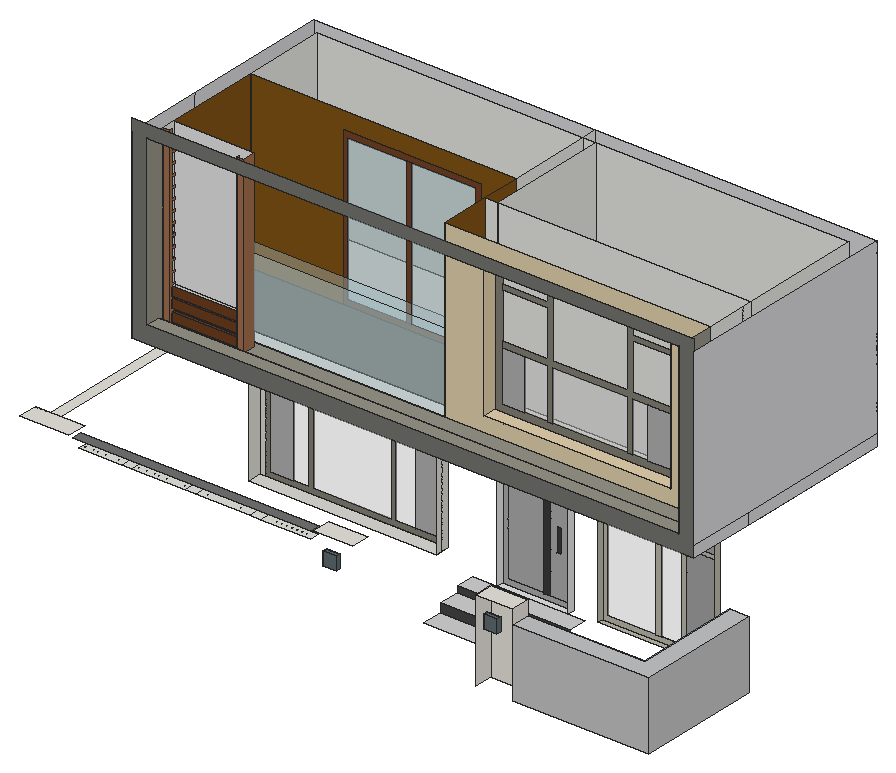
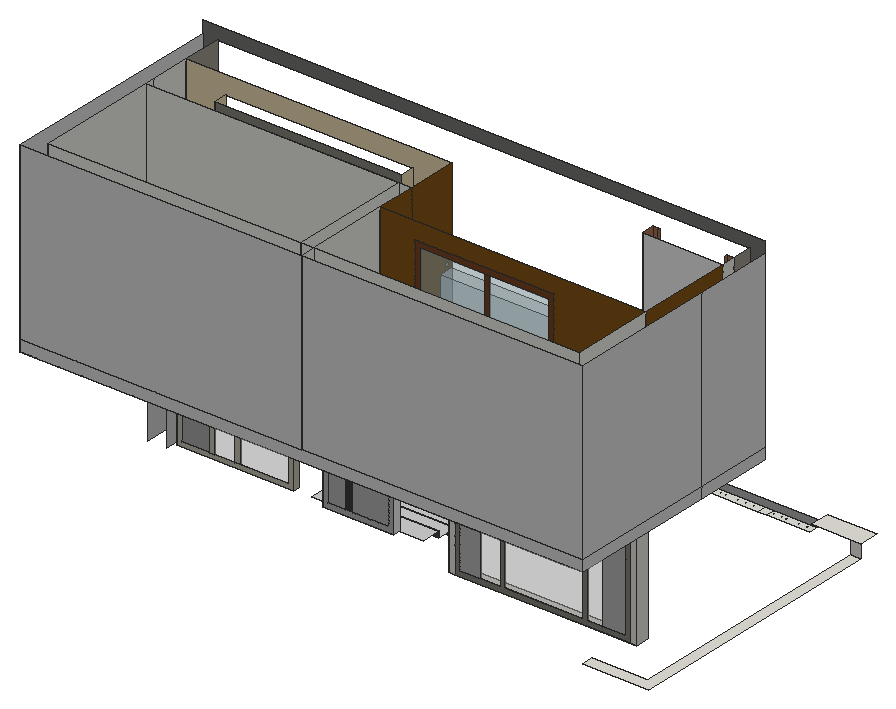
# SketchUp Ruby script. Lengths in inches.
U = 1.inch
M = Sketchup.active_model
def pt(a) = Geom::Point3d.new(a.map { |v| v * U })
def face(e, loops, mat)
  f = e.add_face(loops[0].map { |a| pt(a) })
  loops[1..].each { |l| e.add_face(l.map { |a| pt(a) }).erase! }
  f.material = f.back_material = mat if mat
  f
end
# faces: each face lists its corners as indices into pts; further lists are holes
def faces(e, pts, list, mat = nil) = list.each { |f| face(e, (f[0].is_a?(Array) ? f : [f]).map { |l| l.map { |i| pts[i] } }, mat) }
# xy, xz, yz: faces in a plane at the given z, y or x. An outline is a flat list of corners, or four numbers for a rectangle; further outlines are holes
def ring(l) = l.size == 4 ? [[l[0], l[1]], [l[2], l[1]], [l[2], l[3]], [l[0], l[3]]] : l.each_slice(2).to_a
def flat(e, list, mat, &to3) = list.each { |f| face(e, (f[0].is_a?(Array) ? f : [f]).map { |l| ring(l).map { |u, v| to3.(u, v) } }, mat) }
def xy(e, z, list, mat = nil) = flat(e, list, mat) { |x, y| [x, y, z] }
def xz(e, y, list, mat = nil) = flat(e, list, mat) { |x, z| [x, y, z] }
def yz(e, x, list, mat = nil) = flat(e, list, mat) { |y, z| [x, y, z] }
def lines(e, pts, list) = list.each { |a, b| e.add_line(pt(pts[a]), pt(pts[b])) }
# prism: a flat outline (further loops are holes) pulled along v
def prism(e, loops, v, mat = nil)
  f = face(e, loops, mat); d = Geom::Vector3d.new(v.map { |x| x * U })
  f.pushpull(f.normal.samedirection?(d) ? d.length : -d.length)
end
def box(e, o, s, mat = nil) = prism(e, [[o, [o[0] + s[0], o[1], o[2]], [o[0] + s[0], o[1] + s[1], o[2]], [o[0], o[1] + s[1], o[2]]]], [0, 0, s[2]], mat)
def at(x, y, z, deg = 0) = Geom::Transformation.translation(pt([x, y, z])) * Geom::Transformation.rotation(ORIGIN, Z_AXIS, deg.degrees)
def axes(o, x, y, z) = Geom::Transformation.new([*x, 0, *y, 0, *z, 0, *pt(o).to_a, 1])
def part(name) = M.definitions.add(name)
# library, detail: a bought-in or finely detailed component or shape, given as its bounding box
def library(name, o, s) = part(name).tap { |d| box(d.entities, o, s) }
def detail(e, o, s) = box(e.add_group.entities, o, s)
def put(e, d, t, mat = nil) = e.add_instance(d, t).tap { |i| i.material = mat if mat }
def group(e, t, mat = nil) = e.add_group.tap { |g| g.transformation = t; g.material = mat if mat }.entities
root = M.entities
M.materials.add("[Blinds Vertical Pattern]").color = [212, 212, 214]
M.materials.add("[Blinds Vertical Stripe Gray]").color = [160, 160, 160]
M.materials.add("[Blinds Vertical Stripe Gray]1").color = [175, 175, 175]
M.materials.add("[Blinds Weave]").color = [127, 82, 22]
M.materials.add("[Carpet Diamond Olive]").color = [87, 77, 61]
M.materials.add("[Carrera Marble]").color = [207, 207, 207]
M.materials.add("[Color M01]").color = [226, 226, 226]
M.materials.add("[Color M03]").color = [170, 170, 170]
M.materials.add("[Color M05]").color = [114, 114, 114]
M.materials.add("[Color M07]").color = [58, 58, 58]
M.materials.add("[Concrete Block 8x8 Gray]").color = [114, 114, 111]
M.materials.add("[Fencing Metal Straight]").color = [194, 195, 196]
M.materials.add("[Formica Graystone]").color = [186, 182, 168]
M.materials.add("[Formica Graystone]2").color = [130, 127, 117]
M.materials.add("[Formica Graystone]3").color = [149, 146, 135]
M.materials.add("[Formica Speckled Grey]").color = [94, 105, 111]
M.materials.add("[Granite Dark Gray]").color = [69, 68, 68]
M.materials.add("[Quartz Light Brown]").color = [224, 207, 171]
M.materials.add("[Quartz Light Brown]1").color = [199, 184, 152]
M.materials.add("[Terrazzo Tile Light]").color = [219, 217, 210]
M.materials.add("[Tile Travertine 2 inch]").color = [229, 225, 218]
M.materials.add("[Translucent Glass Gray]").color = [226, 226, 226]
M.materials["[Translucent Glass Gray]"].alpha = 0.5
M.materials.add("[Translucent Glass Gray]1").color = [224, 224, 224]
M.materials["[Translucent Glass Gray]1"].alpha = 0.5
M.materials.add("[Translucent Glass Safety]").color = [179, 206, 214]
M.materials["[Translucent Glass Safety]"].alpha = 0.5
M.materials.add("[Translucent Glass Safety]1").color = [204, 235, 244]
M.materials["[Translucent Glass Safety]1"].alpha = 0.38
M.materials.add("[Wood Cherry Original]").color = [107, 60, 29]
M.materials.add("[Wood Veneer 01]").color = [114, 66, 35]
M.materials.add("[Wood Veneer 02]").color = [160, 108, 76]
xy(root,20.25,[[445.64,200.28,587.08,226.75]],"[Carrera Marble]")
xy(root,31.375,[[445.64,226.75,587.08,253.22]],"[Carrera Marble]")
xy(root,38.0625,[[151.04,291.34,388.47,309.84]],"[Terrazzo Tile Light]")
xy(root,39.19,[[445.64,253.22,587.08,277.72]],"[Carrera Marble]")
xy(root,39.19,[[476.45,277.72,566.07,286.22]],"[Color M01]")
xy(root,43.13,[[604.02,277.72,751.39,284.78]],"[Formica Graystone]")
xy(root,102.5625,[[387.01,114.53,403.76,119.71],[590.2,114.53,606.95,119.71]],"[Formica Speckled Grey]")
xy(root,116.1875,[[622.67,119.71,793.87,119.71,793.87,277.72,769.95,277.72,769.95,143.63,622.67,143.63]],"[Fencing Metal Straight]")
xy(root,116.1875,[[0,143.63,12.5625,143.63,12.5625,464.52,83.3125,464.52,83.3125,479.71,0,479.71]],"[Tile Travertine 2 inch]")
xy(root,119.3125,[[387.01,114.53,403.76,119.71],[590.2,114.53,606.95,119.71]],"[Formica Speckled Grey]")
xy(root,119.59,[[[69.95,125.1875,124.17,137.375],[119.99,129.51,120.39,129.56,120.77,129.72,121.09,129.97,121.34,130.29,121.5,130.67,121.55,131.07,121.5,131.48,121.34,131.86,121.09,132.18,120.77,132.43,120.39,132.58,119.99,132.64,119.59,132.58,119.21,132.43,118.88,132.18,118.64,131.86,118.48,131.48,118.43,131.07,118.48,130.67,118.64,130.29,118.88,129.97,119.21,129.72,119.59,129.56],[115.49,129.51,115.89,129.56,116.27,129.72,116.59,129.97,116.84,130.29,117,130.67,117.05,131.07,117,131.48,116.84,131.86,116.59,132.18,116.27,132.43,115.89,132.58,115.49,132.64,115.09,132.58,114.71,132.43,114.38,132.18,114.14,131.86,113.98,131.48,113.93,131.07,113.98,130.67,114.14,130.29,114.38,129.97,114.71,129.72,115.09,129.56],[110.11,129.51,110.52,129.56,110.9,129.72,111.22,129.97,111.47,130.29,111.625,130.67,111.68,131.07,111.625,131.48,111.47,131.86,111.22,132.18,110.9,132.43,110.52,132.58,110.11,132.64,109.71,132.58,109.33,132.43,109.01,132.18,108.76,131.86,108.61,131.48,108.55,131.07,108.61,130.67,108.76,130.29,109.01,129.97,109.33,129.72,109.71,129.56],[104.36,129.51,104.77,129.56,105.15,129.72,105.47,129.97,105.72,130.29,105.875,130.67,105.93,131.07,105.875,131.48,105.72,131.86,105.47,132.18,105.15,132.43,104.77,132.58,104.36,132.64,103.96,132.58,103.58,132.43,103.26,132.18,103.01,131.86,102.86,131.48,102.8,131.07,102.86,130.67,103.01,130.29,103.26,129.97,103.58,129.72,103.96,129.56],[98.93,129.51,99.33,129.56,99.71,129.72,100.03,129.97,100.28,130.29,100.4375,130.67,100.49,131.07,100.4375,131.48,100.28,131.86,100.03,132.18,99.71,132.43,99.33,132.58,98.93,132.64,98.52,132.58,98.15,132.43,97.82,132.18,97.57,131.86,97.42,131.48,97.36,131.07,97.42,130.67,97.57,130.29,97.82,129.97,98.15,129.72,98.52,129.56],[93.43,129.51,93.83,129.56,94.21,129.72,94.53,129.97,94.78,130.29,94.9375,130.67,94.99,131.07,94.9375,131.48,94.78,131.86,94.53,132.18,94.21,132.43,93.83,132.58,93.43,132.64,93.02,132.58,92.65,132.43,92.32,132.18,92.07,131.86,91.92,131.48,91.86,131.07,91.92,130.67,92.07,130.29,92.32,129.97,92.65,129.72,93.02,129.56],[88.61,129.51,89.02,129.56,89.4,129.72,89.72,129.97,89.97,130.29,90.125,130.67,90.18,131.07,90.125,131.48,89.97,131.86,89.72,132.18,89.4,132.43,89.02,132.58,88.61,132.64,88.21,132.58,87.83,132.43,87.51,132.18,87.26,131.86,87.11,131.48,87.05,131.07,87.11,130.67,87.26,130.29,87.51,129.97,87.83,129.72,88.21,129.56],[83.3,129.51,83.71,129.56,84.08,129.72,84.41,129.97,84.66,130.29,84.8125,130.67,84.86,131.07,84.8125,131.48,84.66,131.86,84.41,132.18,84.08,132.43,83.71,132.58,83.3,132.64,82.9,132.58,82.52,132.43,82.2,132.18,81.95,131.86,81.79,131.48,81.74,131.07,81.79,130.67,81.95,130.29,82.2,129.97,82.52,129.72,82.9,129.56],[78.3,129.51,78.71,129.56,79.08,129.72,79.41,129.97,79.66,130.29,79.8125,130.67,79.86,131.07,79.8125,131.48,79.66,131.86,79.41,132.18,79.08,132.43,78.71,132.58,78.3,132.64,77.9,132.58,77.52,132.43,77.2,132.18,76.95,131.86,76.79,131.48,76.74,131.07,76.79,130.67,76.95,130.29,77.2,129.97,77.52,129.72,77.9,129.56],[73.24,129.51,73.64,129.56,74.02,129.72,74.34,129.97,74.59,130.29,74.75,130.67,74.8,131.07,74.75,131.48,74.59,131.86,74.34,132.18,74.02,132.43,73.64,132.58,73.24,132.64,72.84,132.58,72.46,132.43,72.13,132.18,71.89,131.86,71.73,131.48,71.68,131.07,71.73,130.67,71.89,130.29,72.13,129.97,72.46,129.72,72.84,129.56]],[124.17,125.1875,136.24,137.375],[[136.24,125.1875,204.36,137.375],[198.68,129.51,199.08,129.56,199.46,129.72,199.78,129.97,200.03,130.29,200.1875,130.67,200.24,131.07,200.1875,131.48,200.03,131.86,199.78,132.18,199.46,132.43,199.08,132.58,198.68,132.64,198.27,132.58,197.9,132.43,197.57,132.18,197.32,131.86,197.17,131.48,197.11,131.07,197.17,130.67,197.32,130.29,197.57,129.97,197.9,129.72,198.27,129.56],[193.18,129.51,193.58,129.56,193.96,129.72,194.28,129.97,194.53,130.29,194.6875,130.67,194.74,131.07,194.6875,131.48,194.53,131.86,194.28,132.18,193.96,132.43,193.58,132.58,193.18,132.64,192.77,132.58,192.4,132.43,192.07,132.18,191.82,131.86,191.67,131.48,191.61,131.07,191.67,130.67,191.82,130.29,192.07,129.97,192.4,129.72,192.77,129.56],[187.68,129.51,188.08,129.56,188.46,129.72,188.78,129.97,189.03,130.29,189.1875,130.67,189.24,131.07,189.1875,131.48,189.03,131.86,188.78,132.18,188.46,132.43,188.08,132.58,187.68,132.64,187.27,132.58,186.9,132.43,186.57,132.18,186.32,131.86,186.17,131.48,186.11,131.07,186.17,130.67,186.32,130.29,186.57,129.97,186.9,129.72,187.27,129.56],[181.18,129.51,181.58,129.56,181.96,129.72,182.28,129.97,182.53,130.29,182.6875,130.67,182.74,131.07,182.6875,131.48,182.53,131.86,182.28,132.18,181.96,132.43,181.58,132.58,181.18,132.64,180.77,132.58,180.4,132.43,180.07,132.18,179.82,131.86,179.67,131.48,179.61,131.07,179.67,130.67,179.82,130.29,180.07,129.97,180.4,129.72,180.77,129.56],[176.11,129.51,176.52,129.56,176.9,129.72,177.22,129.97,177.47,130.29,177.625,130.67,177.68,131.07,177.625,131.48,177.47,131.86,177.22,132.18,176.9,132.43,176.52,132.58,176.11,132.64,175.71,132.58,175.33,132.43,175.01,132.18,174.76,131.86,174.61,131.48,174.55,131.07,174.61,130.67,174.76,130.29,175.01,129.97,175.33,129.72,175.71,129.56],[171.05,129.51,171.46,129.56,171.83,129.72,172.16,129.97,172.41,130.29,172.5625,130.67,172.61,131.07,172.5625,131.48,172.41,131.86,172.16,132.18,171.83,132.43,171.46,132.58,171.05,132.64,170.65,132.58,170.27,132.43,169.95,132.18,169.7,131.86,169.54,131.48,169.49,131.07,169.54,130.67,169.7,130.29,169.95,129.97,170.27,129.72,170.65,129.56],[165.99,129.51,166.39,129.56,166.77,129.72,167.09,129.97,167.34,130.29,167.5,130.67,167.55,131.07,167.5,131.48,167.34,131.86,167.09,132.18,166.77,132.43,166.39,132.58,165.99,132.64,165.59,132.58,165.21,132.43,164.88,132.18,164.64,131.86,164.48,131.48,164.43,131.07,164.48,130.67,164.64,130.29,164.88,129.97,165.21,129.72,165.59,129.56],[160.93,129.51,161.33,129.56,161.71,129.72,162.03,129.97,162.28,130.29,162.4375,130.67,162.49,131.07,162.4375,131.48,162.28,131.86,162.03,132.18,161.71,132.43,161.33,132.58,160.93,132.64,160.52,132.58,160.15,132.43,159.82,132.18,159.57,131.86,159.42,131.48,159.36,131.07,159.42,130.67,159.57,130.29,159.82,129.97,160.15,129.72,160.52,129.56],[155.86,129.51,156.27,129.56,156.65,129.72,156.97,129.97,157.22,130.29,157.375,130.67,157.43,131.07,157.375,131.48,157.22,131.86,156.97,132.18,156.65,132.43,156.27,132.58,155.86,132.64,155.46,132.58,155.08,132.43,154.76,132.18,154.51,131.86,154.36,131.48,154.3,131.07,154.36,130.67,154.51,130.29,154.76,129.97,155.08,129.72,155.46,129.56],[150.8,129.51,151.21,129.56,151.58,129.72,151.91,129.97,152.16,130.29,152.3125,130.67,152.36,131.07,152.3125,131.48,152.16,131.86,151.91,132.18,151.58,132.43,151.21,132.58,150.8,132.64,150.4,132.58,150.02,132.43,149.7,132.18,149.45,131.86,149.29,131.48,149.24,131.07,149.29,130.67,149.45,130.29,149.7,129.97,150.02,129.72,150.4,129.56],[145.74,129.51,146.14,129.56,146.52,129.72,146.84,129.97,147.09,130.29,147.25,130.67,147.3,131.07,147.25,131.48,147.09,131.86,146.84,132.18,146.52,132.43,146.14,132.58,145.74,132.64,145.34,132.58,144.96,132.43,144.63,132.18,144.39,131.86,144.23,131.48,144.18,131.07,144.23,130.67,144.39,130.29,144.63,129.97,144.96,129.72,145.34,129.56],[140.68,129.51,141.08,129.56,141.46,129.72,141.78,129.97,142.03,130.29,142.1875,130.67,142.24,131.07,142.1875,131.48,142.03,131.86,141.78,132.18,141.46,132.43,141.08,132.58,140.68,132.64,140.27,132.58,139.9,132.43,139.57,132.18,139.32,131.86,139.17,131.48,139.11,131.07,139.17,130.67,139.32,130.29,139.57,129.97,139.9,129.72,140.27,129.56]],[204.36,125.1875,217.93,137.375],[[217.93,125.1875,285.42,137.375],[280.86,129.51,281.27,129.56,281.65,129.72,281.97,129.97,282.22,130.29,282.375,130.67,282.43,131.07,282.375,131.48,282.22,131.86,281.97,132.18,281.65,132.43,281.27,132.58,280.86,132.64,280.46,132.58,280.08,132.43,279.76,132.18,279.51,131.86,279.36,131.48,279.3,131.07,279.36,130.67,279.51,130.29,279.76,129.97,280.08,129.72,280.46,129.56],[275.43,129.51,275.83,129.56,276.21,129.72,276.53,129.97,276.78,130.29,276.9375,130.67,276.99,131.07,276.9375,131.48,276.78,131.86,276.53,132.18,276.21,132.43,275.83,132.58,275.43,132.64,275.02,132.58,274.65,132.43,274.32,132.18,274.07,131.86,273.92,131.48,273.86,131.07,273.92,130.67,274.07,130.29,274.32,129.97,274.65,129.72,275.02,129.56],[269.74,129.51,270.14,129.56,270.52,129.72,270.84,129.97,271.09,130.29,271.25,130.67,271.3,131.07,271.25,131.48,271.09,131.86,270.84,132.18,270.52,132.43,270.14,132.58,269.74,132.64,269.34,132.58,268.96,132.43,268.63,132.18,268.39,131.86,268.23,131.48,268.18,131.07,268.23,130.67,268.39,130.29,268.63,129.97,268.96,129.72,269.34,129.56],[264.74,129.51,265.14,129.56,265.52,129.72,265.84,129.97,266.09,130.29,266.25,130.67,266.3,131.07,266.25,131.48,266.09,131.86,265.84,132.18,265.52,132.43,265.14,132.58,264.74,132.64,264.34,132.58,263.96,132.43,263.63,132.18,263.39,131.86,263.23,131.48,263.18,131.07,263.23,130.67,263.39,130.29,263.63,129.97,263.96,129.72,264.34,129.56],[259.18,129.51,259.58,129.56,259.96,129.72,260.28,129.97,260.53,130.29,260.6875,130.67,260.74,131.07,260.6875,131.48,260.53,131.86,260.28,132.18,259.96,132.43,259.58,132.58,259.18,132.64,258.77,132.58,258.4,132.43,258.07,132.18,257.82,131.86,257.67,131.48,257.61,131.07,257.67,130.67,257.82,130.29,258.07,129.97,258.4,129.72,258.77,129.56],[251.86,129.51,252.27,129.56,252.65,129.72,252.97,129.97,253.22,130.29,253.375,130.67,253.43,131.07,253.375,131.48,253.22,131.86,252.97,132.18,252.65,132.43,252.27,132.58,251.86,132.64,251.46,132.58,251.08,132.43,250.76,132.18,250.51,131.86,250.36,131.48,250.3,131.07,250.36,130.67,250.51,130.29,250.76,129.97,251.08,129.72,251.46,129.56],[244.99,129.51,245.39,129.56,245.77,129.72,246.09,129.97,246.34,130.29,246.5,130.67,246.55,131.07,246.5,131.48,246.34,131.86,246.09,132.18,245.77,132.43,245.39,132.58,244.99,132.64,244.59,132.58,244.21,132.43,243.88,132.18,243.64,131.86,243.48,131.48,243.43,131.07,243.48,130.67,243.64,130.29,243.88,129.97,244.21,129.72,244.59,129.56],[239.24,129.51,239.64,129.56,240.02,129.72,240.34,129.97,240.59,130.29,240.75,130.67,240.8,131.07,240.75,131.48,240.59,131.86,240.34,132.18,240.02,132.43,239.64,132.58,239.24,132.64,238.84,132.58,238.46,132.43,238.13,132.18,237.89,131.86,237.73,131.48,237.68,131.07,237.73,130.67,237.89,130.29,238.13,129.97,238.46,129.72,238.84,129.56],[233.24,129.51,233.64,129.56,234.02,129.72,234.34,129.97,234.59,130.29,234.75,130.67,234.8,131.07,234.75,131.48,234.59,131.86,234.34,132.18,234.02,132.43,233.64,132.58,233.24,132.64,232.84,132.58,232.46,132.43,232.13,132.18,231.89,131.86,231.73,131.48,231.68,131.07,231.73,130.67,231.89,130.29,232.13,129.97,232.46,129.72,232.84,129.56],[227.8,129.51,228.21,129.56,228.58,129.72,228.91,129.97,229.16,130.29,229.3125,130.67,229.36,131.07,229.3125,131.48,229.16,131.86,228.91,132.18,228.58,132.43,228.21,132.58,227.8,132.64,227.4,132.58,227.02,132.43,226.7,132.18,226.45,131.86,226.29,131.48,226.24,131.07,226.29,130.67,226.45,130.29,226.7,129.97,227.02,129.72,227.4,129.56],[222.24,129.51,222.64,129.56,223.02,129.72,223.34,129.97,223.59,130.29,223.75,130.67,223.8,131.07,223.75,131.48,223.59,131.86,223.34,132.18,223.02,132.43,222.64,132.58,222.24,132.64,221.84,132.58,221.46,132.43,221.13,132.18,220.89,131.86,220.73,131.48,220.68,131.07,220.73,130.67,220.89,130.29,221.13,129.97,221.46,129.72,221.84,129.56]],
  [285.42,125.1875,299.8,137.375],[[299.8,125.1875,362.74,137.375],[358.68,129.51,359.08,129.56,359.46,129.72,359.78,129.97,360.03,130.29,360.1875,130.67,360.24,131.07,360.1875,131.48,360.03,131.86,359.78,132.18,359.46,132.43,359.08,132.58,358.68,132.64,358.27,132.58,357.9,132.43,357.57,132.18,357.32,131.86,357.17,131.48,357.11,131.07,357.17,130.67,357.32,130.29,357.57,129.97,357.9,129.72,358.27,129.56],[353.05,129.51,353.46,129.56,353.83,129.72,354.16,129.97,354.41,130.29,354.5625,130.67,354.61,131.07,354.5625,131.48,354.41,131.86,354.16,132.18,353.83,132.43,353.46,132.58,353.05,132.64,352.65,132.58,352.27,132.43,351.95,132.18,351.7,131.86,351.54,131.48,351.49,131.07,351.54,130.67,351.7,130.29,351.95,129.97,352.27,129.72,352.65,129.56],[347.05,129.51,347.46,129.56,347.83,129.72,348.16,129.97,348.41,130.29,348.5625,130.67,348.61,131.07,348.5625,131.48,348.41,131.86,348.16,132.18,347.83,132.43,347.46,132.58,347.05,132.64,346.65,132.58,346.27,132.43,345.95,132.18,345.7,131.86,345.54,131.48,345.49,131.07,345.54,130.67,345.7,130.29,345.95,129.97,346.27,129.72,346.65,129.56],[340.86,129.51,341.27,129.56,341.65,129.72,341.97,129.97,342.22,130.29,342.375,130.67,342.43,131.07,342.375,131.48,342.22,131.86,341.97,132.18,341.65,132.43,341.27,132.58,340.86,132.64,340.46,132.58,340.08,132.43,339.76,132.18,339.51,131.86,339.36,131.48,339.3,131.07,339.36,130.67,339.51,130.29,339.76,129.97,340.08,129.72,340.46,129.56],[334.49,129.51,334.89,129.56,335.27,129.72,335.59,129.97,335.84,130.29,336,130.67,336.05,131.07,336,131.48,335.84,131.86,335.59,132.18,335.27,132.43,334.89,132.58,334.49,132.64,334.09,132.58,333.71,132.43,333.38,132.18,333.14,131.86,332.98,131.48,332.93,131.07,332.98,130.67,333.14,130.29,333.38,129.97,333.71,129.72,334.09,129.56],[327.61,129.51,328.02,129.56,328.4,129.72,328.72,129.97,328.97,130.29,329.125,130.67,329.18,131.07,329.125,131.48,328.97,131.86,328.72,132.18,328.4,132.43,328.02,132.58,327.61,132.64,327.21,132.58,326.83,132.43,326.51,132.18,326.26,131.86,326.11,131.48,326.05,131.07,326.11,130.67,326.26,130.29,326.51,129.97,326.83,129.72,327.21,129.56],[321.55,129.51,321.96,129.56,322.33,129.72,322.66,129.97,322.91,130.29,323.0625,130.67,323.11,131.07,323.0625,131.48,322.91,131.86,322.66,132.18,322.33,132.43,321.96,132.58,321.55,132.64,321.15,132.58,320.77,132.43,320.45,132.18,320.2,131.86,320.04,131.48,319.99,131.07,320.04,130.67,320.2,130.29,320.45,129.97,320.77,129.72,321.15,129.56],[315.49,129.51,315.89,129.56,316.27,129.72,316.59,129.97,316.84,130.29,317,130.67,317.05,131.07,317,131.48,316.84,131.86,316.59,132.18,316.27,132.43,315.89,132.58,315.49,132.64,315.09,132.58,314.71,132.43,314.38,132.18,314.14,131.86,313.98,131.48,313.93,131.07,313.98,130.67,314.14,130.29,314.38,129.97,314.71,129.72,315.09,129.56],[309.68,129.51,310.08,129.56,310.46,129.72,310.78,129.97,311.03,130.29,311.1875,130.67,311.24,131.07,311.1875,131.48,311.03,131.86,310.78,132.18,310.46,132.43,310.08,132.58,309.68,132.64,309.27,132.58,308.9,132.43,308.57,132.18,308.32,131.86,308.17,131.48,308.11,131.07,308.17,130.67,308.32,130.29,308.57,129.97,308.9,129.72,309.27,129.56],[303.86,129.51,304.27,129.56,304.65,129.72,304.97,129.97,305.22,130.29,305.375,130.67,305.43,131.07,305.375,131.48,305.22,131.86,304.97,132.18,304.65,132.43,304.27,132.58,303.86,132.64,303.46,132.58,303.08,132.43,302.76,132.18,302.51,131.86,302.36,131.48,302.3,131.07,302.36,130.67,302.51,130.29,302.76,129.97,303.08,129.72,303.46,129.56]]])
xy(root,128.625,[[61.88,125.1875,362.74,137.375],[362.74,125.1875,371.37,137.375]],"[Color M05]")
xy(root,133.9375,[[0,119.71,61.88,143.63],[371.37,119.71,419.6875,143.63],[575.77,119.71,622.67,143.63]],"[Tile Travertine 2 inch]")
xy(root,192.07,[[476.45,277.72,566.07,286.22]],"[Color M01]")
xy(root,199.88,[[604.02,277.72,751.39,284.78]],"[Formica Graystone]")
xy(root,220,[[438.59,277.72,769.95,291.34],[769.95,277.72,793.87,291.34],[83.3125,291.34,107.23,479.71],[107.23,291.34,151.04,309.84],[388.47,291.34,438.59,309.84],
  [438.59,291.34,769.95,299.71],[769.95,291.34,793.87,299.71],[438.59,299.71,769.95,309.84],[769.95,299.71,793.87,309.84],[107.23,309.84,438.59,479.71],
  [438.59,309.84,769.95,455.8],[769.95,309.84,793.87,479.71],[438.59,455.8,769.95,479.71]])
xy(root,220,[[83.3125,191.84,83.3125,291.34,151.04,291.34,151.04,309.84,388.47,309.84,388.47,291.34,438.59,291.34,438.59,277.72,793.87,277.72,793.87,191.84]],"[Quartz Light Brown]1")
xy(root,233.875,[[102.3,217.06,102.3,233.68,204.43,233.68,204.43,217.06,195.83,217.06,195.83,224.74,110.71,224.74,110.71,217.06],[102.3,241.34,438.59,258.82],[438.59,241.34,774.88,305.05],[438.59,305.05,455.13,460.72],[455.13,305.05,774.88,460.72],
  [102.3,355.28,438.59,460.72]])
xy(root,233.875,[[102.3,258.82,438.59,355.28]],"[Carpet Diamond Olive]")
xy(root,233.875,[[102.3,210.84,774.88,210.84,774.88,241.34,102.3,241.34,102.3,233.68,204.43,233.68,204.43,217.06,195.83,217.06,195.83,224.74,110.71,224.74,110.71,217.06,102.3,217.06]],"[Formica Graystone]3")
xy(root,235.58,[[110.71,220.49,195.02,224.74],[195.02,220.49,195.83,224.74]])
xy(root,240.875,[[102.3,191.84,774.88,210.84]],"[Formica Graystone]3")
xy(root,246.5625,[[110.71,220.49,195.83,224.74]],"[Wood Cherry Original]")
xy(root,251.21,[[110.71,220.49,195.02,224.74],[195.02,220.49,195.83,224.74]],"[Wood Cherry Original]")
xy(root,252.34,[[488.69,241.34,724.51,258.97]],"[Quartz Light Brown]")
xy(root,262.1875,[[110.71,220.49,195.83,224.74]],"[Wood Cherry Original]")
xy(root,264.96,[[110.71,220.49,195.02,224.74],[195.02,220.49,195.83,224.74]],"[Wood Cherry Original]")
xz(root,114.53,[[387.01,102.5625,403.76,119.3125],[590.2,102.5625,606.95,119.3125]],"[Formica Speckled Grey]")
xz(root,119.71,[[622.67,30.25,793.87,116.1875]],"[Fencing Metal Straight]")
xz(root,119.71,[[387.01,102.5625,403.76,119.3125],[590.2,102.5625,606.95,119.3125]],"[Tile Travertine 2 inch]")
xz(root,143.63,[[622.67,30.25,769.95,116.1875]],"[Fencing Metal Straight]")
xz(root,143.63,[[575.77,30.25,622.67,133.9375],[0,116.1875,12.5625,133.9375]],"[Tile Travertine 2 inch]")
xz(root,191.84,[[[83.3125,220,793.87,468.5],[102.3,240.875,774.88,453.4375]]],"[Concrete Block 8x8 Gray]")
xz(root,210.84,[[102.3,233.875,774.88,240.875]])
xz(root,217.06,[[102.3,233.875,110.71,453.4375],[195.83,233.875,204.43,453.4375]],"[Wood Veneer 02]")
xz(root,220.49,[[110.71,235.58,195.83,246.5625],[110.71,251.21,195.83,262.1875],[110.71,264.96,195.83,275.9375]],"[Wood Cherry Original]")
xz(root,224.74,[[110.71,233.875,195.83,235.58],[110.71,235.58,195.83,246.5625],[110.71,251.21,195.83,262.1875],[110.71,264.96,195.83,275.9375]])
xz(root,224.74,[[110.71,246.5625,195.83,251.21],[110.71,262.1875,195.83,264.96]],"[Color M07]")
xz(root,226.75,[[445.64,20.25,587.08,31.375]],"[Granite Dark Gray]")
xz(root,233.68,[[102.3,233.875,204.43,453.4375]],"[Color M01]")
xz(root,241.34,[[[438.59,233.875,774.88,453.4375],[488.69,252.34,724.51,430]]],"[Quartz Light Brown]")
xz(root,241.34,[[102.3,233.875,438.59,334.75]],"[Translucent Glass Safety]1")
xz(root,253.22,[[445.64,31.375,587.08,39.19]],"[Granite Dark Gray]")
xz(root,258.82,[[102.3,233.875,438.59,334.75]],"[Translucent Glass Safety]1")
xz(root,258.97,[[497.89,261.53,526.43,324.32],[682.12,261.53,715.3125,324.32]],"[Blinds Vertical Stripe Gray]1")
xz(root,258.97,[[[488.69,252.34,724.51,430],[497.89,261.53,715.3125,420.81]],[554.98,261.53,561.48,261.53,561.48,324.32,656.23,324.32,656.23,261.53,662.73,261.53,662.73,324.32,715.3125,324.32,715.3125,332.38,662.73,332.38,662.73,390.39,715.3125,390.39,715.3125,396.84,662.73,396.84,662.73,420.81,656.23,420.81,656.23,332.38,561.48,332.38,561.48,420.81,554.98,420.81,554.98,396.84,497.89,396.84,497.89,390.39,554.98,390.39,554.98,332.38,497.89,332.38,497.89,324.32,554.98,324.32]],"[Formica Graystone]2")
xz(root,258.97,[[526.43,261.53,554.98,324.32],[561.48,261.53,656.23,324.32],[662.73,261.53,682.12,324.32]],"[Translucent Glass Gray]1")
xz(root,284.78,[[709.83,49.33,745.2,160.38],[709.83,166.1875,745.2,193.69]],"[Blinds Vertical Stripe Gray]")
xz(root,284.78,[[[604.02,43.13,751.39,199.88],[610.21,49.33,745.2,193.69]],[703.5,49.33,709.83,49.33,709.83,160.38,745.2,160.38,745.2,166.1875,709.83,166.1875,709.83,193.69,703.5,193.69,703.5,166.1875,610.21,166.1875,610.21,160.38,703.5,160.38],[671.48,49.33,678.13,160.38]],"[Formica Graystone]")
xz(root,284.78,[[610.21,49.33,671.48,160.38],[678.13,49.33,703.5,160.38],[610.21,166.1875,703.5,193.69]],"[Translucent Glass Gray]")
xz(root,286.22,[[[476.45,39.19,566.07,192.07],[482.78,45.53,559.74,185.73]],[482.78,45.53,528.93,185.73],[[536.82,45.53,559.74,185.73],[544.4,97.47,550.84,127.72]]],"[Color M03]")
xz(root,286.22,[[528.93,45.53,536.82,185.73],[544.4,97.47,550.84,127.72]],"[Color M07]")
xz(root,305.05,[[438.59,233.875,455.13,453.4375],[455.13,233.875,774.88,453.4375]])
xz(root,309.84,[[165.125,44.66,194.04,163.12],[348.27,44.66,373.92,163.12],[165.125,168.44,194.04,194.09],[348.27,168.44,373.92,194.09]],"[Blinds Vertical Stripe Gray]1")
xz(root,309.84,[[[158.52,38.0625,380.52,200.6875],[165.125,44.66,165.125,163.12,213.14,163.12,213.14,44.66,218.37,44.66,218.37,163.12,317.39,163.12,317.39,44.66,322.62,44.66,322.62,163.12,373.92,163.12,373.92,168.44,322.62,168.44,322.62,194.09,317.39,194.09,317.39,168.44,218.37,168.44,218.37,194.09,213.14,194.09,213.14,168.44,165.125,168.44,165.125,194.09,373.92,194.09,373.92,44.66]]],"[Formica Graystone]2")
xz(root,309.84,[[151.04,38.0625,158.52,38.0625,158.52,200.6875,380.52,200.6875,380.52,38.0625,388.47,38.0625,388.47,220,151.04,220]],"[Terrazzo Tile Light]")
xz(root,309.84,[[194.04,44.66,213.14,163.12],[218.37,44.66,317.39,163.12],[322.62,44.66,348.27,163.12],[194.04,168.44,213.14,194.09],[218.37,168.44,317.39,194.09],
  [322.62,168.44,348.27,194.09]],"[Translucent Glass Gray]")
xz(root,355.28,[[102.3,233.875,218.57,233.875,218.57,432.125,395.07,432.125,395.07,233.875,438.59,233.875,438.59,453.4375,102.3,453.4375]],"[Blinds Weave]")
xz(root,355.28,[[225.9375,241.25,299.82,424.75],[306.71,241.25,387.7,424.75]],"[Translucent Glass Safety]")
xz(root,355.28,[[[218.57,233.875,395.07,432.125],[225.9375,241.25,387.7,424.75]],[299.82,241.25,306.71,424.75]],"[Wood Veneer 01]")
xz(root,460.72,[[102.3,233.875,438.59,453.4375],[438.59,233.875,455.13,453.4375],[455.13,233.875,774.88,453.4375]])
xz(root,479.71,[[83.3125,220,793.87,233.875],[83.3125,233.875,438.59,453.4375],[438.59,233.875,793.87,453.4375]],"[Blinds Vertical Pattern]")
yz(root,83.3125,[[191.84,220,291.34,233.875],[291.34,220,479.71,233.875],[191.84,233.875,291.34,453.4375],[291.34,233.875,479.71,453.4375]],"[Blinds Vertical Pattern]")
yz(root,102.3,[[217.06,233.875,233.68,453.4375],[241.34,233.875,258.82,334.75],[355.28,233.875,460.72,453.4375]])
yz(root,102.3,[[[233.68,233.875,241.34,233.875,241.34,334.75,258.82,334.75,258.82,233.875,355.28,233.875,355.28,453.4375,233.68,453.4375],[250.08,339.44,249.34,339.54,248.64,339.83,248.05,340.28,247.59,340.88,247.3,341.57,247.21,342.32,247.3,343.06,247.59,343.75,248.05,344.35,248.64,344.81,249.34,345.09,250.08,345.19,250.83,345.09,251.52,344.81,252.11,344.35,252.57,343.75,252.86,343.06,252.96,342.32,252.86,341.57,252.57,340.88,252.11,340.28,251.52,339.83,250.83,339.54]]],"[Blinds Weave]")
yz(root,102.3,[[210.84,233.875,217.06,233.875,217.06,453.4375,191.84,453.4375,191.84,240.875,210.84,240.875]],"[Formica Graystone]3")
yz(root,110.71,[[220.49,235.58,224.74,246.5625],[220.49,251.21,224.74,262.1875],[220.49,264.96,224.74,275.9375]])
yz(root,110.71,[[217.06,233.875,224.74,233.875,224.74,235.58,220.49,235.58,220.49,246.5625,224.74,246.5625,224.74,251.21,220.49,251.21,220.49,262.1875,224.74,262.1875,224.74,264.96,220.49,264.96,220.49,275.9375,224.74,275.9375,224.74,278.71,220.49,278.71,220.49,289.6875,224.74,289.6875,224.74,292.46,220.49,292.46,220.49,303.4375,224.74,303.4375,224.74,306.21,220.49,306.21,220.49,317.1875,224.74,317.1875,224.74,319.83,220.49,319.83,220.49,330.8125,224.74,330.8125,224.74,333.46,220.49,333.46,220.49,344.4375,224.74,344.4375,224.74,347.08,220.49,347.08,220.49,358.0625,224.74,358.0625,224.74,360.71,220.49,360.71,220.49,371.6875,224.74,371.6875,224.74,374.33,220.49,374.33,220.49,385.3125,224.74,385.3125,224.74,387.96,220.49,387.96,220.49,398.9375,224.74,398.9375,224.74,401.58,220.49,401.58,220.49,412.5625,224.74,412.5625,224.74,415.21,220.49,415.21,220.49,426.1875,224.74,426.1875,224.74,428.83,220.49,428.83,220.49,439.8125,224.74,439.8125,224.74,442.46,220.49,442.46,220.49,453.4375,217.06,453.4375]],"[Wood Veneer 02]")
yz(root,151.04,[[291.34,38.0625,309.84,220]],"[Terrazzo Tile Light]")
yz(root,195.83,[[220.49,235.58,224.74,246.5625],[220.49,251.21,224.74,262.1875],[220.49,264.96,224.74,275.9375]])
yz(root,195.83,[[217.06,233.875,217.06,453.4375,220.49,453.4375,220.49,442.46,224.74,442.46,224.74,439.8125,220.49,439.8125,220.49,428.83,224.74,428.83,224.74,426.1875,220.49,426.1875,220.49,415.21,224.74,415.21,224.74,412.5625,220.49,412.5625,220.49,401.58,224.74,401.58,224.74,398.9375,220.49,398.9375,220.49,387.96,224.74,387.96,224.74,385.3125,220.49,385.3125,220.49,374.33,224.74,374.33,224.74,371.6875,220.49,371.6875,220.49,360.71,224.74,360.71,224.74,358.0625,220.49,358.0625,220.49,347.08,224.74,347.08,224.74,344.4375,220.49,344.4375,220.49,333.46,224.74,333.46,224.74,330.8125,220.49,330.8125,220.49,319.83,224.74,319.83,224.74,317.1875,220.49,317.1875,220.49,306.21,224.74,306.21,224.74,303.4375,220.49,303.4375,220.49,292.46,224.74,292.46,224.74,289.6875,220.49,289.6875,220.49,278.71,224.74,278.71,224.74,275.9375,220.49,275.9375,220.49,264.96,224.74,264.96,224.74,262.1875,220.49,262.1875,220.49,251.21,224.74,251.21,224.74,246.5625,220.49,246.5625,220.49,235.58,224.74,235.58,224.74,233.875]],"[Wood Veneer 02]")
yz(root,204.43,[[217.06,233.875,233.68,453.4375]],"[Wood Veneer 02]")
yz(root,387.01,[[114.53,102.5625,119.71,119.3125]],"[Formica Speckled Grey]")
yz(root,388.47,[[291.34,38.0625,299.71,220],[299.71,38.0625,309.84,220]],"[Terrazzo Tile Light]")
yz(root,403.76,[[114.53,102.5625,119.71,119.3125]],"[Formica Speckled Grey]")
yz(root,438.59,[[241.34,233.875,258.82,334.75],[355.28,233.875,460.72,453.4375],[460.72,233.875,479.71,453.4375]])
yz(root,438.59,[[[258.82,233.875,258.82,334.75,241.34,334.75,241.34,453.4375,305.05,453.4375,305.05,233.875],[250.08,339.44,250.83,339.54,251.52,339.83,252.11,340.28,252.57,340.88,252.86,341.57,252.96,342.32,252.86,343.06,252.57,343.75,252.11,344.35,251.52,344.81,250.83,345.09,250.08,345.19,249.34,345.09,248.64,344.81,248.05,344.35,247.59,343.75,247.3,343.06,247.21,342.32,247.3,341.57,247.59,340.88,248.05,340.28,248.64,339.83,249.34,339.54]],[305.05,233.875,355.28,453.4375]],"[Blinds Weave]")
yz(root,455.13,[[305.05,233.875,460.72,453.4375]])
yz(root,476.45,[[277.72,39.19,286.22,192.07]],"[Color M01]")
yz(root,488.69,[[241.34,252.34,258.97,430]],"[Quartz Light Brown]")
yz(root,566.07,[[277.72,39.19,286.22,192.07]],"[Color M01]")
yz(root,575.77,[[119.71,30.25,143.63,133.9375]],"[Tile Travertine 2 inch]")
yz(root,590.2,[[114.53,102.5625,119.71,119.3125]],"[Formica Speckled Grey]")
yz(root,604.02,[[277.72,43.13,284.78,199.88]],"[Formica Graystone]")
yz(root,606.95,[[114.53,102.5625,119.71,119.3125]],"[Formica Speckled Grey]")
yz(root,622.67,[[119.71,116.1875,143.63,133.9375]],"[Tile Travertine 2 inch]")
yz(root,724.51,[[241.34,252.34,258.97,430]],"[Quartz Light Brown]")
yz(root,751.39,[[277.72,43.13,284.78,199.88]],"[Formica Graystone]")
yz(root,769.95,[[143.63,30.25,277.72,116.1875]],"[Fencing Metal Straight]")
yz(root,774.88,[[241.34,233.875,292.25,453.4375],[292.25,233.875,305.05,453.4375],[305.05,233.875,460.72,453.4375]])
yz(root,774.88,[[210.84,233.875,210.84,240.875,191.84,240.875,191.84,453.4375,241.34,453.4375,241.34,233.875]],"[Formica Graystone]3")
yz(root,793.87,[[191.84,220,277.72,233.875],[277.72,220,479.71,233.875],[191.84,233.875,479.71,453.4375]],"[Blinds Vertical Pattern]")
yz(root,793.87,[[119.71,30.25,277.72,116.1875]],"[Fencing Metal Straight]")
